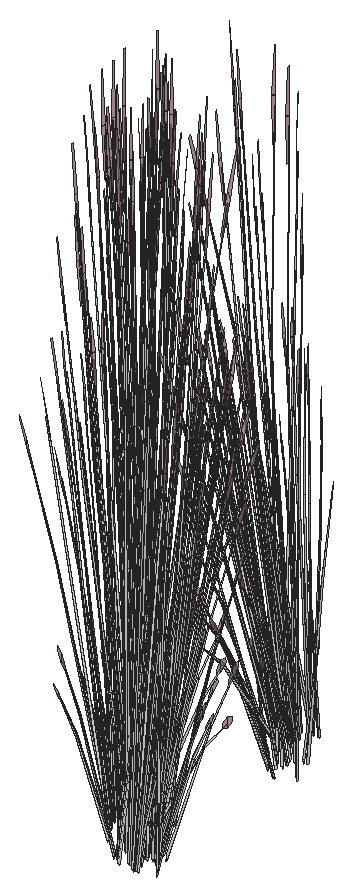
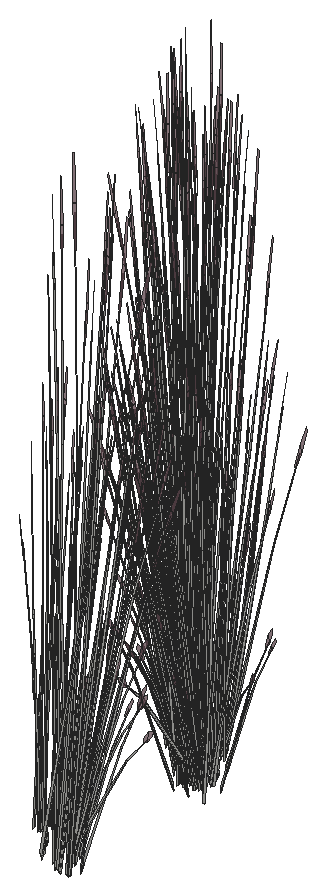
# SketchUp Ruby script. Lengths in inches.
U = 1.inch
M = Sketchup.active_model
def pt(a) = Geom::Point3d.new(a.map { |v| v * U })
def face(e, loops, mat)
  f = e.add_face(loops[0].map { |a| pt(a) })
  loops[1..].each { |l| e.add_face(l.map { |a| pt(a) }).erase! }
  f.material = f.back_material = mat if mat
  f
end
# faces: each face lists its corners as indices into pts; further lists are holes
def faces(e, pts, list, mat = nil) = list.each { |f| face(e, (f[0].is_a?(Array) ? f : [f]).map { |l| l.map { |i| pts[i] } }, mat) }
# xy, xz, yz: faces in a plane at the given z, y or x. An outline is a flat list of corners, or four numbers for a rectangle; further outlines are holes
def ring(l) = l.size == 4 ? [[l[0], l[1]], [l[2], l[1]], [l[2], l[3]], [l[0], l[3]]] : l.each_slice(2).to_a
def flat(e, list, mat, &to3) = list.each { |f| face(e, (f[0].is_a?(Array) ? f : [f]).map { |l| ring(l).map { |u, v| to3.(u, v) } }, mat) }
def xy(e, z, list, mat = nil) = flat(e, list, mat) { |x, y| [x, y, z] }
def xz(e, y, list, mat = nil) = flat(e, list, mat) { |x, z| [x, y, z] }
def yz(e, x, list, mat = nil) = flat(e, list, mat) { |y, z| [x, y, z] }
def lines(e, pts, list) = list.each { |a, b| e.add_line(pt(pts[a]), pt(pts[b])) }
# prism: a flat outline (further loops are holes) pulled along v
def prism(e, loops, v, mat = nil)
  f = face(e, loops, mat); d = Geom::Vector3d.new(v.map { |x| x * U })
  f.pushpull(f.normal.samedirection?(d) ? d.length : -d.length)
end
def box(e, o, s, mat = nil) = prism(e, [[o, [o[0] + s[0], o[1], o[2]], [o[0] + s[0], o[1] + s[1], o[2]], [o[0], o[1] + s[1], o[2]]]], [0, 0, s[2]], mat)
def at(x, y, z, deg = 0) = Geom::Transformation.translation(pt([x, y, z])) * Geom::Transformation.rotation(ORIGIN, Z_AXIS, deg.degrees)
def axes(o, x, y, z) = Geom::Transformation.new([*x, 0, *y, 0, *z, 0, *pt(o).to_a, 1])
def part(name) = M.definitions.add(name)
# library, detail: a bought-in or finely detailed component or shape, given as its bounding box
def library(name, o, s) = part(name).tap { |d| box(d.entities, o, s) }
def detail(e, o, s) = box(e.add_group.entities, o, s)
def put(e, d, t, mat = nil) = e.add_instance(d, t).tap { |i| i.material = mat if mat }
def group(e, t, mat = nil) = e.add_group.tap { |g| g.transformation = t; g.material = mat if mat }.entities
root = M.entities
M.materials.add("LightPink_Translucent").color = [144, 107, 117]
M.materials["LightPink_Translucent"].alpha = 0.75
c1 = part("blade")
p = [[2.15,0.21,22],[0,0.17,0],[0.09,0.45,0],[2.18,0.31,22],[2.29,0.31,22],[0.38,0.45,0],
  [2.48,0.24,33],[2.49,0.24,33],[2.48,0.22,33]]
faces(c1.entities,p,[[0,1,2,3],[4,5,2,3],[6,3,4,7],[8,0,3,6]])
c2 = part("seeds")
p = [[0.3,-0.1,1.38],[-0.01,-0.03,1.59],[-0.01,-0.03,0.03],[0.14,-0.07,-0.07],[0.29,-0.03,3],[0.15,0.01,3.11]]
faces(c2.entities,p,[[0,1,2,3],[1,0,4,5]],"LightPink_Translucent")
c3 = part("blade with seeds")
put(c3.entities,c1,at(0,0,0))
put(c3.entities,c2,axes([2.4,0.25,30.99],[1.5799,-0.05474,1.17369],[-0.12525,1.92788,0.29478],[-0.07173,-0.02425,1.56792]))
put(root,c3,axes([329.78,500.37,1402.68],[-0.25628,0.30892,-0.51099],[-0.22444,-0.32634,-0.3958],[-0.13021,-0.047,0.97773]))
put(root,c3,axes([329.97,500.23,1403.05],[0.20082,0.29199,0.35414],[-0.2293,0.2764,-0.4572],[-0.1165,-0.04206,0.87481]))
put(root,c3,axes([329.2,500.78,1400.77],[0.22533,-0.03337,1.1486],[-0.14293,0.29403,0.84392],[-0.11135,-0.04411,0.25299]))
put(root,c3,axes([330.79,501.05,1400.72],[-0.38326,0.02879,0.44739],[-0.03466,-0.47788,-0.21531],[0.06861,-0.04843,1.43643]))
put(root,c3,axes([329.91,500.05,1403.03],[-0.0189,0.47427,-0.1216],[-0.35781,-0.01296,-0.67495],[-0.13781,-0.03295,1.02557]))
put(root,c3,axes([329.8,501.4,1400.48],[0,0.46636,0.49651],[-0.39487,0,0],[0,-0.10622,1.57504]))
put(root,c3,axes([332.59,501.87,1403.03],[-0.17758,-0.42229,-0.1216],[0.31518,-0.20752,-0.67495],[0.13282,-0.05572,1.02557]))
put(root,c3,axes([332.57,501.51,1402.68],[0.09562,-0.42421,-0.51099],[0.32782,0.1454,-0.3958],[0.13199,-0.0389,0.97773]))
put(root,c3,axes([332.06,499.78,1400.375],[0.22066,-0.46731,0],[0.36918,0.26061,-0.51607],[0.08408,0.05936,1.63711]))
put(root,c3,axes([329.46,500.7,1401.875],[0.14639,-0.01056,1.71376],[-0.09712,0.45778,0.13857],[-0.20862,-0.02831,0.73262]))
put(root,c3,axes([330.73,501.78,1400.21],[-0.21202,-0.39143,-0.44739],[0.32115,-0.27564,0.21531],[-0.06861,-0.04843,1.43643]))
put(root,c3,axes([330.78,501.23,1400.36],[0.15345,0.52148,0.45755],[-0.43845,0.18134,0.17955],[0.00536,-0.09582,1.58856]))
put(root,c3,axes([332.92,501.625,1399.98],[-0.22732,0.05597,1.41583],[-0.03618,-0.44548,0.08104],[0.15921,-0.06743,0.80566]))
put(root,c3,axes([333.34,501.23,1400.26],[-0.21881,-0.29821,-0.06488],[0.23965,-0.27324,-0.29416],[0.0679,-0.01924,0.97024]))
put(root,c3,axes([330.7,501.64,1400.72],[-0.17124,0.42022,0.44739],[-0.35581,-0.20224,-0.21531],[0,-0.09687,1.43643]))
put(root,c3,axes([331.33,501.27,1400.21],[0,-0.53961,0],[0.44133,0,0],[0,0,1.79456]))
put(root,c3,axes([331.87,500.02,1400.48],[-0.33032,-0.23318,0.49651],[0.19744,-0.41812,0],[0.07523,0.05311,1.57504]))
put(root,c3,axes([332.51,501.66,1402.98],[0.31014,-0.20596,-0.71045],[0.17284,0.42397,0.08574],[0.14985,-0.04816,1.00501]))
put(root,c3,axes([330.54,501.93,1400.06],[-0.36714,-0.07646,-0.62353],[0.07747,-0.47163,-0.16365],[-0.10956,-0.05715,1.37633]))
put(root,c3,axes([331.12,500.93,1400.36],[-0.29264,0.42323,0.45755],[-0.34767,-0.3736,0.17955],[0.07055,-0.04224,1.58856]))
put(root,c3,axes([331.44,501.6875,1400.3],[-0.32829,-0.4014,-0.06131],[0.32849,-0.40164,0],[-0.01146,-0.01402,1.75571]))
put(root,c3,axes([330.61,500.23,1400.47],[-0.10196,0.46348,0.17642],[-0.3731,-0.13116,0.35086],[0.06445,-0.00226,1.60407]))
put(root,c3,axes([332.47,501.74,1403.05],[-0.29332,-0.1301,0.35414],[0.08555,-0.37955,-0.4572],[0.11809,-0.0348,0.87481]))
put(root,c3,axes([329.4,501.05,1402.73],[0.09971,-0.42522,0.48003],[0.32782,0.1454,0.3958],[-0.12892,0.02555,0.9933]))
put(root,c3,axes([330.46,500.61,1399.59],[-0.3474,0.18671,1.28929],[-0.11057,-0.53572,0.50096],[0.21332,0.00891,1.46642]))
put(root,c3,axes([331.39,500.75,1400.62],[0.06809,-0.4162,0.1448],[0.33266,0.07225,-0.41347],[0.06054,0.04274,1.26744]))
put(root,c3,axes([329.37,500.9375,1402.73],[-0.12963,-0.31798,0.0643],[0.23638,-0.15564,0.50621],[-0.1042,0.03071,0.77189]))
put(root,c3,axes([330.82,501.74,1400.36],[0.44609,0.09826,0.45755],[-0.09078,0.55493,0.17955],[-0.06519,-0.05359,1.58856]))
put(root,c3,axes([333.17,501.33,1399.49],[-0.01845,-0.0708,1.76342],[0.12793,-0.41416,-0.26939],[0.12905,-0.00596,0.30037]))
put(root,c3,axes([329.36,501.26,1399.49],[0.00895,0.0735,1.76342],[-0.18044,0.38382,-0.26939],[-0.12817,-0.01935,0.30037]))
put(root,c3,axes([331.25,500.86,1400.72],[-0.21202,-0.39143,0.44739],[0.32115,-0.27564,-0.21531],[0.06861,0.04843,1.43643]))
put(root,c3,axes([330.15,502.65,1400.03],[-0.08291,-0.40636,-0.30978],[0.32928,-0.11539,0.30978],[-0.06638,-0.04686,1.38974]))
put(root,c3,axes([330.58,502.625,1400.47],[0.37926,-0.12378,0.17642],[0.09365,0.46065,0.35086],[-0.03382,-0.06712,1.60407]))
put(root,c3,axes([331.36,500.88,1400.67],[0.35635,-0.30962,-0.29095],[0.23697,0.43749,-0.50002],[0.08792,0.04443,1.59708]))
put(root,c3,axes([332.78,501.7,1402.53],[0.29332,0.1301,-0.35414],[-0.08555,0.37955,0.4572],[0.11809,-0.0348,0.87481]))
put(root,c3,axes([330.0625,502.82,1400.02],[-0.33032,-0.23318,-0.49651],[0.19744,-0.41812,0],[-0.07523,-0.05311,1.57504]))
put(root,c3,axes([332.26,500.0625,1400.02],[0.33032,0.23318,-0.49651],[-0.19744,0.41812,0],[0.07523,0.05311,1.57504]))
put(root,c3,axes([329.33,501.1,1402.53],[-0.29332,-0.1301,-0.35414],[0.08555,-0.37955,0.4572],[-0.11809,0.0348,0.87481]))
put(root,c3,axes([331.63,501.39,1400.21],[0.39487,0,0],[0,0.48281,0],[0,0,1.78407]))
put(root,c3,axes([330.96,502,1400.67],[-0.35635,0.30962,-0.29095],[-0.23697,-0.43749,-0.50002],[-0.08792,-0.04443,1.59708]))
put(root,c3,axes([331.74,500.26,1400.47],[-0.37926,0.12378,0.17642],[-0.09365,-0.46065,0.35086],[0.03382,0.06712,1.60407]))
put(root,c3,axes([331.98,501.23,1401.875],[-0.14639,0.01056,1.71376],[0.09712,-0.45778,0.13857],[0.20862,0.02831,0.73262]))
put(root,c3,axes([332.17,500.23,1400.03],[0.08291,0.40636,-0.30978],[-0.32928,0.11539,0.30978],[0.06638,0.04686,1.38974]))
put(root,c3,axes([332.73,501.86,1402.73],[0.12963,0.31798,0.0643],[-0.23638,0.15564,0.50621],[0.1042,-0.03071,0.77189]))
put(root,c3,axes([331.5,501.15,1400.38],[-0.44609,-0.09826,0.49198],[0.09078,-0.55493,0.19306],[0.06519,0.05359,1.70813]))
put(root,c3,axes([332.71,501.75,1402.73],[-0.09971,0.42522,0.48003],[-0.32782,-0.1454,0.3958],[0.12892,-0.02555,0.9933]))
put(root,c3,axes([331.15,502.52,1400.2],[-0.11516,-0.40207,0],[0.32884,-0.1408,0],[0,0,1.54371]))
put(root,c3,axes([330.93,502.13,1400.62],[-0.06809,0.4162,0.1448],[-0.33266,-0.07225,-0.41347],[-0.06054,-0.04274,1.26744]))
put(root,c3,axes([329.64,501.05,1403.05],[0.29332,0.1301,0.35414],[-0.08555,0.37955,-0.4572],[-0.11809,0.0348,0.87481]))
put(root,c3,axes([331.58,502.46,1400.18],[0.37054,-0.15823,-0.19198],[0.1302,0.45581,0.00008],[0.0409,-0.01749,1.73897]))
put(root,c3,axes([331.71,502.65,1400.47],[0.10196,-0.46348,0.17642],[0.3731,0.13116,0.35086],[-0.06445,0.00226,1.60407]))
put(root,c3,axes([331.62,501.6,1400.21],[0.24637,0.30123,0],[-0.24637,0.30123,0],[0,0,1.69266]))
put(root,c3,axes([330.22,501.03,1401.34],[0.10032,-0.06746,1.77064],[0.0346,0.47103,0.13857],[-0.2173,0.0625,0.63284]))
put(root,c3,axes([332.29,501.47,1400.47],[-0.2773,-0.3397,0.17642],[0.27945,-0.32949,0.35086],[-0.03063,0.06937,1.60407]))
put(root,c3,axes([331.78,500.95,1400.06],[0.36714,0.07646,-0.62353],[-0.07747,0.47163,-0.16365],[0.10956,0.05715,1.37633]))
put(root,c3,axes([333.4,501.78,1400.77],[-0.21807,0.07699,1.1486],[0.10265,-0.31819,0.84392],[0.11568,0.02177,0.25299]))
put(root,c3,axes([331.07,502.7,1400.2],[-0.35581,-0.20937,0],[0.17124,-0.43505,0],[0,0,1.62707]))
put(root,c3,axes([331.36,502.14,1400.46],[-0.34464,-0.37536,-0.25192],[0.29,-0.42149,0.5513],[-0.0928,0.04391,1.68216]))
put(root,c3,axes([330.45,502.86,1400.48],[0.33032,0.23318,0.49651],[-0.19744,0.41812,0],[-0.07523,-0.05311,1.57504]))
put(root,c3,axes([331.62,501.25,1400.72],[0.17124,-0.42022,0.44739],[0.35581,0.20224,-0.21531],[0,0.09687,1.43643]))
put(root,c3,axes([333.3,503.125,1402.71],[-0.03191,-0.04083,1.77383],[0.06981,-0.43764,-0.16761],[0.12571,-0.02796,0.31391]))
put(root,c3,axes([329.14,501.35,1402.72],[-0.05763,0.06055,1.74944],[0.0049,0.44239,-0.27667],[-0.13211,0.05753,0.14031]))
put(root,c3,axes([331.55,501.49,1400.29],[0,0.53934,-0.05637],[-0.44133,0,0],[0,0.01695,1.79368]))
put(root,c3,axes([329.53,501.29,1402.68],[-0.09562,0.42421,-0.51099],[-0.32782,-0.1454,-0.3958],[-0.13199,0.0389,0.97773]))
put(root,c3,axes([329.51,500.93,1403.03],[0.17758,0.42229,-0.1216],[-0.31518,0.20752,-0.67495],[-0.13282,0.05572,1.02557]))
put(root,c3,axes([331.58,501.1,1400.21],[0.21202,0.39143,-0.44739],[-0.32115,0.27564,0.21531],[0.06861,0.04843,1.43643]))
put(root,c3,axes([333.02,502.76,1401.93],[-0.06755,-0.39203,-0.03492],[0.31928,-0.09013,-0.15832],[0.06667,0.02485,0.52218]))
put(root,c3,axes([330.26,503.1,1400.375],[-0.22066,0.46731,0],[-0.36918,-0.26061,-0.51607],[-0.08408,-0.05936,1.63711]))
put(root,c3,axes([332.19,502.75,1403.03],[0.0189,-0.47427,-0.1216],[0.35781,0.01296,-0.67495],[0.13781,0.03295,1.02557]))
put(root,c3,axes([332.52,501.48,1400.48],[0,-0.46636,0.49651],[0.39487,0,0],[0,0.10622,1.57504]))
put(root,c3,axes([331.53,501.83,1400.72],[0.38326,-0.02879,0.44739],[0.03466,0.47788,-0.21531],[-0.06861,0.04843,1.43643]))
put(root,c3,axes([331.77,501.34,1400.62],[0.32884,-0.136,0.1448],[0.11516,0.38837,-0.41347],[0,0.08547,1.26744]))
put(root,c3,axes([332.14,502.5625,1403.05],[-0.20082,-0.29199,0.35414],[0.2293,-0.2764,-0.4572],[0.1165,0.04206,0.87481]))
put(root,c3,axes([331.1875,502.06,1400.21],[-0.38326,0.02879,-0.44739],[-0.03466,-0.47788,0.21531],[-0.06861,0.04843,1.43643]))
put(root,c3,axes([332.99,502.29,1400.59],[-0.085,-0.1147,1.43002],[0.1106,-0.37943,-0.30754],[0.17198,0.0514,0.61141]))
put(root,c3,axes([331.47,502.71,1400.2],[0.35581,0.20937,0],[-0.17124,0.43505,0],[0,0,1.74954]))
put(root,c3,axes([332.5,502.46,1402.72],[0.07571,-0.00789,1.74944],[0.20767,-0.36231,-0.27667],[0.13467,0.04783,0.14031]))
put(root,c3,axes([331.61,503.17,1400.19],[-0.21791,-0.46895,-0.05142],[0.36918,-0.26061,0.51607],[-0.09097,0.04465,1.6363]))
put(root,c3,axes([331.53,502.03,1400.62],[0.26075,0.2802,0.1448],[-0.2175,0.31612,-0.41347],[-0.06054,0.04274,1.26744]))
put(root,c3,axes([329.47,502.11,1402.73],[-0.08753,-0.42921,0.48003],[0.34336,-0.07449,0.3958],[-0.1012,0.10094,0.9933]))
put(root,c3,axes([329.41,502.03,1402.73],[-0.2423,-0.19613,0.0643],[0.14107,-0.2793,0.50621],[-0.07768,0.0903,0.77189]))
put(root,c3,axes([329.52,501.51,1401.875],[0.12246,-0.09864,1.71376],[0.1031,0.45582,0.13857],[-0.19225,0.10302,0.73262]))
put(root,c3,axes([332.21,502.52,1402.98],[0.35281,0.01123,-0.71045],[-0.0237,0.47284,0.08574],[0.14947,0.0499,1.00501]))
put(root,c3,axes([331.8125,502.9,1400.48],[0.33032,-0.23318,0.49651],[0.19744,0.41812,0],[-0.07523,0.05311,1.57504]))
put(root,c3,axes([331.34,502.53,1400.29],[0.15345,0.53576,-0.06012],[-0.43845,0.18773,0],[0.00536,0.01871,1.72173]))
put(root,c3,axes([331.51,503.11,1400.03],[-0.32928,-0.11539,-0.30978],[0.08291,-0.40636,0.30978],[-0.06638,0.04686,1.38974]))
put(root,c3,axes([329.14,502.28,1400.59],[0.12266,0.03828,1.43002],[0.07906,0.39104,-0.30754],[-0.16661,0.0732,0.61141]))
put(root,c3,axes([329.6875,501.96,1403.05],[0.30722,-0.06665,0.35414],[0.08112,0.381,-0.4572],[-0.08804,0.10234,0.87481]))
put(root,c3,axes([332.78,501.56,1400.375],[0.44133,0,0],[0,0.52122,-0.51607],[0,0.11871,1.63711]))
put(root,c3,axes([328.5,501.8,1402.71],[0.04504,0.01251,1.77383],[0.13934,0.41205,-0.16761],[-0.0922,0.10815,0.31391]))
put(root,c3,axes([332.61,501.83,1400.2],[-0.44111,-0.00373,-0.04976],[0,-0.52122,0.49943],[-0.01386,0.11865,1.58352]))
put(root,c3,axes([331.65,501.375,1400.67],[0.39748,0.22252,-0.29095],[-0.19139,0.46966,-0.50002],[0.01249,0.11531,1.59708]))
put(root,c3,axes([328.88,503.1,1400.77],[0.14709,-0.21136,1.1486],[0.05804,0.3346,0.84392],[-0.1063,0.05991,0.25299]))
put(root,c3,axes([332.42,502.71,1402.53],[0.20082,0.29199,-0.35414],[-0.2293,0.2764,0.4572],[0.1165,0.04206,0.87481]))
put(root,c3,axes([332.52,501.9,1400.03],[-0.24637,0.29097,-0.30978],[-0.24637,-0.29097,0.30978],[0,0.09372,1.38974]))
put(root,c3,axes([331.46,501.93,1400.67],[0.04113,0.53214,-0.29095],[-0.42835,0.03218,-0.50002],[-0.07543,0.07088,1.59708]))
put(root,c3,axes([332.32,502.83,1402.73],[-0.01777,0.35463,0.0643],[-0.26836,-0.00972,0.50621],[0.1028,0.03711,0.77189]))
put(root,c3,axes([331.61,501.72,1400.21],[-0.17124,0.42022,-0.44739],[-0.35581,-0.20224,0.21531],[0,0.09687,1.43643]))
put(root,c3,axes([329.43,502.19,1402.53],[-0.30722,0.06665,-0.35414],[-0.08112,-0.381,0.4572],[-0.08804,0.10234,0.87481]))
put(root,c3,axes([332.34,502.71,1402.73],[-0.26024,0.30729,0.48003],[-0.22444,-0.32634,0.3958],[0.1221,0.05668,0.9933]))
put(root,c3,axes([328.99,503.05,1403.65],[0.31145,0.12449,-0.06488],[-0.0958,0.38314,-0.29416],[-0.05094,0.05817,0.97024]))
put(root,c3,axes([331.2,502.34,1400.06],[-0.23773,0.35053,-0.62353],[-0.29532,-0.31785,-0.16365],[-0.09526,0.08744,1.37633]))
put(root,c3,axes([331.52,503.07,1403.05],[-0.05451,-0.37564,0.35414],[0.31161,-0.09919,-0.4572],[0.0837,0.10765,0.87481]))
put(root,c3,axes([331.62,502.93,1400.33],[0.44186,0.15158,0.30756],[-0.11054,0.54181,-0.36492],[-0.07313,0.06781,1.64885]))
put(root,c3,axes([331.59,503.29,1400.02],[-0.33032,0.23318,-0.49651],[-0.19744,-0.41812,0],[-0.07523,0.05311,1.57504]))
put(root,c3,axes([332.6875,501.91,1400.02],[0,0.46636,-0.49651],[-0.39487,0,0],[0,0.10622,1.57504]))
put(root,c3,axes([331.7,501.97,1401.875],[-0.1311,-0.08035,1.71376],[0.27131,-0.33708,0.13857],[0.16909,0.15206,0.73262]))
put(root,c3,axes([331.72,500.91,1402.47],[-0.30498,-0.24231,1.38283],[0.32203,-0.37727,0.59665],[0.0984,0.22736,1.33663]))
put(root,c3,axes([329.53,501.93,1403.03],[0.32648,0.25715,-0.1216],[-0.18809,0.3724,-0.67495],[-0.09224,0.12945,1.02557]))
put(root,c3,axes([332.18,502.88,1400.77],[-0.19872,-0.13409,1.1486],[0.2566,-0.13625,0.84392],[0.06921,0.11541,0.25299]))
put(root,c3,axes([331.49,503.26,1403.03],[0.21031,-0.39918,-0.1216],[0.30457,0.22997,-0.67495],[0.10587,0.11278,1.02557]))
put(root,c3,axes([329.97,501.82,1401.875],[0.08815,-0.14329,1.71376],[0.22258,0.38678,0.13857],[-0.15267,0.17614,0.73262]))
put(root,c3,axes([329.6875,502.23,1402.68],[0.09067,0.42583,-0.51099],[-0.34336,0.07449,-0.3958],[-0.0984,0.11438,0.97773]))
put(root,c3,axes([330.1,502.72,1403.05],[0.23881,-0.24554,0.35414],[0.22606,0.28036,-0.4572],[-0.0344,0.14245,0.87481]))
put(root,c3,axes([331.89,503.22,1400.375],[0.22066,0.46731,0],[-0.36918,0.26061,-0.51607],[-0.08408,0.05936,1.63711]))
put(root,c3,axes([331.21,503.59,1402.71],[0.00104,-0.05646,1.77383],[0.30246,-0.2491,-0.16761],[0.10506,0.08891,0.31391]))
put(root,c3,axes([332.24,503.38,1399.49],[0.02571,-0.06733,1.76342],[0.32373,-0.19829,-0.26939],[0.09815,0.10263,0.30037]))
put(root,c3,axes([331.7,501.37,1400.84],[-0.00964,-0.43909,1.41272],[0.43635,0.11382,0.59816],[-0.1032,0.24027,1.3335]))
put(root,c3,axes([331.8125,501.85,1400.09],[0.12941,0.42699,-0.69212],[-0.37279,0.15378,-0.18165],[0.0143,0.14459,1.52773]))
put(root,c3,axes([329.88,502.95,1402.73],[-0.29004,-0.02173,0.0643],[0.00795,-0.32812,0.50621],[-0.03035,0.12569,0.77189]))
put(root,c3,axes([329.27,503.32,1399.49],[0.04734,0.04659,1.76342],[0.08027,0.4317,-0.26939],[-0.10492,0.09206,0.30037]))
put(root,c3,axes([329.98,502.98,1402.73],[-0.25132,-0.3182,0.48003],[0.2669,-0.27442,0.3958],[-0.04636,0.14929,0.9933]))
put(root,c3,axes([331.74,503.06,1402.68],[0.34827,-0.11086,-0.51099],[0.06092,0.41983,-0.3958],[0.09354,0.12031,0.97773]))
put(root,c3,axes([330.77,503.13,1403.05],[0.1064,-0.35863,0.35414],[0.31043,0.1046,-0.4572],[0.02846,0.14439,0.87481]))
put(root,c3,axes([332.22,503.49,1400.67],[-0.22633,-0.01463,1.0506],[0.14947,-0.31064,0.58006],[0.08941,0.11036,0.8241]))
put(root,c3,axes([331.56,503.41,1402.73],[-0.16041,0.29625,0.0643],[-0.22843,-0.17248,0.50621],[0.07385,0.09498,0.77189]))
put(root,c3,axes([331.1875,504.41,1403.65],[0.2439,-0.26754,-0.06488],[0.22348,0.29302,-0.29416],[0.01573,0.08303,0.97024]))
put(root,c3,axes([331.63,503.33,1402.73],[-0.35104,0.10702,0.48003],[-0.06092,-0.41983,0.3958],[0.08256,0.12373,0.9933]))
put(root,c3,axes([329.9,502.17,1401.875],[0.06572,-0.16029,1.71376],[0.27569,0.33172,0.13857],[-0.12437,0.20675,0.73262]))
put(root,c3,axes([331.48,502.74,1400.59],[0.00623,-0.15459,1.43002],[0.29764,-0.17268,-0.30754],[0.09188,0.18503,0.61141]))
put(root,c3,axes([330.67,503.45,1402.73],[-0.26007,0.1585,0.0643],[-0.12729,-0.28902,0.50621],[0.02512,0.1274,0.77189]))
put(root,c3,axes([329.98,503.07,1402.53],[-0.23881,0.24554,-0.35414],[-0.22606,-0.28036,0.4572],[-0.0344,0.14245,0.87481]))
put(root,c3,axes([329.15,503,1402.72],[-0.00877,0.09229,1.74944],[0.24897,0.32105,-0.27667],[-0.06518,0.15182,0.14031]))
put(root,c3,axes([329.95,502.79,1403.4],[0.3879,0.02311,-0.13498],[-0.0106,0.43749,-0.74919],[-0.02694,0.1685,1.13838]))
put(root,c3,axes([330.67,503.28,1403.03],[0.34538,-0.21713,-0.1216],[0.16972,0.38536,-0.67495],[0.04557,0.16239,1.02557]))
put(root,c3,axes([330.77,503.42,1403.0625],[-0.34777,-0.12192,0.53283],[0.11892,-0.40083,0.43934],[0.0209,0.15763,1.10256]))
put(root,c3,axes([330.13,504.03,1400.77],[-0.00913,-0.2773,1.1486],[0.22824,0.19778,0.84392],[-0.04489,0.13217,0.25299]))
put(root,c3,axes([330.73,503.36,1399.49],[0.05712,-0.02538,1.76342],[0.34359,0.13968,-0.26939],[0.01005,0.15742,0.30037]))
put(root,c3,axes([330.21,502.96,1403],[0.25266,0.31335,-0.5672],[-0.2669,0.27442,-0.43934],[-0.03844,0.15921,1.08528]))
put(root,c3,axes([329.9375,503.43,1400.82],[0.32063,-0.08258,0.06507],[0.07371,0.33271,-0.86304],[-0.02033,0.16842,0.7736]))
put(root,c3,axes([330.96,503.26,1402.68],[0.34695,0.11691,-0.51099],[-0.11892,0.40083,-0.3958],[0.03181,0.16138,0.97773]))
put(root,c3,axes([331.16,502.43,1401.875],[-0.08068,-0.14973,1.71376],[0.3728,-0.12606,0.13857],[0.08426,0.23506,0.73262]))
put(root,c3,axes([330.8,503.51,1402.53],[-0.1064,0.35863,-0.35414],[-0.31043,-0.1046,0.4572],[0.02846,0.14439,0.87481]))
put(root,c3,axes([330.13,502.8125,1403.34],[-0.00918,0.43138,-0.7886],[-0.38672,-0.02897,0.09517],[-0.04081,0.18275,1.11556]))
put(root,c3,axes([329.125,503.95,1402.71],[0.04004,-0.02816,1.77383],[0.33095,0.18728,-0.16761],[-0.00778,0.15594,0.31391]))
put(root,c3,axes([330.5,502.51,1401.875],[-0.00864,-0.17899,1.71376],[0.37441,0.11874,0.13857],[-0.02316,0.25508,0.73262]))
put(root,c3,axes([330.84,503.18,1402.98],[0.16845,0.3792,-0.71045],[-0.34676,0.21133,0.08574],[0.03939,0.18322,1.00501]))
put(root,c3,axes([329.86,503.78,1400.59],[0.11138,-0.07357,1.43002],[0.27499,0.22183,-0.30754],[-0.08185,0.19194,0.61141]))
put(root,c3,axes([330.58,504.14,1402.72],[0.04474,0.0751,1.74944],[0.36104,0.0295,-0.27667],[0.03631,0.16562,0.14031]))
put(root,c3,axes([330.01,503.42,1401.36],[0.00775,-0.24075,1.54345],[0.34877,0.12716,0.21329],[-0.03022,0.25658,0.72882]))
put(root,c3,axes([330.27,517.78,1401.875],[0.08068,0.14973,1.71376],[-0.3728,0.12606,0.13857],[-0.08426,-0.23506,0.73262]))
put(root,c3,axes([330.89,516.79,1402.72],[-0.05398,-0.06539,1.74944],[-0.36026,0.04145,-0.27667],[-0.0575,-0.15639,0.14031]))
put(root,c3,axes([331.72,517.5625,1400.59],[-0.10032,0.0944,1.43002],[-0.30046,-0.16522,-0.30754],[0.05569,-0.20547,0.61141]))
put(root,c3,axes([331.27,517.89,1402.98],[-0.16845,-0.3792,-0.71045],[0.34676,-0.21133,0.08574],[-0.03939,-0.18322,1.00501]))
put(root,c3,axes([330.17,517.38,1400.59],[-0.02137,0.15256,1.43002],[-0.31245,0.12771,-0.30754],[-0.07303,-0.19719,0.61141]))
put(root,c3,axes([330.98,517.05,1399.49],[-0.0592,0.0168,1.76342],[-0.32738,-0.18913,-0.26939],[0.00549,-0.15776,0.30037]))
put(root,c3,axes([331.97,518.26,1402.98],[0.00918,-0.43138,-0.71045],[0.38672,0.02897,0.08574],[0.04081,-0.18275,1.00501]))
put(root,c3,axes([332.51,517.59,1402.72],[-0.00341,-0.09282,1.74944],[-0.28775,-0.26825,-0.27667],[0.04449,-0.16261,0.14031]))
put(root,c3,axes([331.3,517.57,1402.53],[0.1064,-0.35863,-0.35414],[0.31043,0.1046,0.4572],[-0.02846,-0.14439,0.87481]))
put(root,c3,axes([331.53,518.04,1401.875],[-0.06572,0.16029,1.71376],[-0.27569,-0.33172,0.13857],[0.12437,-0.20675,0.73262]))
put(root,c3,axes([332.43,517.25,1402.71],[-0.03584,0.03562,1.77383],[-0.35118,-0.12018,-0.16761],[-0.01271,-0.15545,0.31391]))
put(root,c3,axes([331.14,517.8125,1402.68],[-0.34695,-0.11691,-0.51099],[0.11892,-0.40083,-0.3958],[-0.03181,-0.16138,0.97773]))
put(root,c3,axes([331.35,516.81,1400.77],[0.04528,0.27194,1.1486],[-0.25117,-0.15062,0.84392],[0.02703,-0.13924,0.25299]))
put(root,c3,axes([331.89,518.12,1402.68],[-0.25266,-0.31335,-0.51099],[0.2669,-0.27442,-0.3958],[0.03844,-0.15921,0.97773]))
put(root,c3,axes([330.52,516.57,1402.71],[-0.00658,0.0559,1.77383],[-0.32474,0.20287,-0.16761],[-0.09556,-0.1037,0.31391]))
put(root,c3,axes([330.45,517.5625,1403.09],[0.39316,-0.11987,0.53763],[0.06823,0.47021,0.4433],[-0.09247,-0.13858,1.11249]))
put(root,c3,axes([331.34,517.65,1402.73],[0.34777,0.12192,0.48003],[-0.11892,0.40083,0.3958],[-0.0209,-0.15763,0.9933]))
put(root,c3,axes([331.4375,517.79,1403.03],[-0.34538,0.21713,-0.1216],[-0.16972,-0.38536,-0.67495],[-0.04557,-0.16239,1.02557]))
put(root,c3,axes([332.15,518.28,1403.03],[-0.3879,-0.02311,-0.1216],[0.0106,-0.43749,-0.67495],[0.02694,-0.1685,1.02557]))
put(root,c3,axes([332.13,518,1402.53],[0.23881,-0.24554,-0.35414],[0.22606,0.28036,0.4572],[0.0344,-0.14245,0.87481]))
put(root,c3,axes([330.0625,517.14,1400.77],[0.18411,0.16231,1.1486],[-0.26813,0.09757,0.84392],[-0.05737,-0.12474,0.25299]))
put(root,c3,axes([331.43,517.62,1402.73],[0.26007,-0.1585,0.0643],[0.12729,0.28902,0.50621],[-0.02512,-0.1274,0.77189]))
put(root,c3,axes([330.51,518,1402.98],[-0.30095,-0.22541,-0.71045],[0.21388,-0.395,0.08574],[-0.10904,-0.13459,1.00501]))
put(root,c3,axes([330.4,517.7,1402.53],[-0.05451,-0.37564,-0.35414],[0.31161,-0.09919,0.4572],[-0.0837,-0.10765,0.87481]))
put(root,c3,axes([330.54,517.66,1402.73],[0.16041,-0.29625,0.0643],[0.22843,0.17248,0.50621],[-0.07385,-0.09498,0.77189]))
put(root,c3,axes([329.92,517.625,1399.49],[-0.03419,0.06144,1.76342],[-0.3455,0.13246,-0.26939],[-0.08346,-0.12049,0.30037]))
put(root,c3,axes([330.49,519.3125,1400.1],[-0.14494,-0.47823,-0.69835],[0.41752,-0.17223,-0.18329],[-0.01602,-0.16194,1.54149]))
put(root,c3,axes([329.73,518.25,1401.875],[0.1311,0.08035,1.71376],[-0.27131,0.33708,0.13857],[-0.16909,-0.15206,0.73262]))
put(root,c3,axes([332.43,517.85,1399.49],[-0.05283,-0.03674,1.76342],[-0.13569,-0.41045,-0.26939],[0.09154,-0.11138,0.30037]))
put(root,c3,axes([331.33,517.95,1403.05],[-0.1064,0.35863,0.35414],[-0.31043,-0.1046,-0.4572],[-0.02846,-0.14439,0.87481]))
put(root,c3,axes([330.37,518.01,1402.68],[-0.34827,0.11086,-0.51099],[-0.06092,-0.41983,-0.3958],[-0.09354,-0.12031,0.97773]))
put(root,c3,axes([332.125,518.1,1402.73],[0.25132,0.3182,0.48003],[-0.2669,0.27442,0.3958],[0.04636,-0.14929,0.9933]))
put(root,c3,axes([330.61,517.63,1403.43],[-0.23555,0.44708,-0.13619],[-0.34112,-0.25757,-0.75594],[-0.11858,-0.12631,1.14864]))
put(root,c3,axes([332.22,518.125,1402.73],[0.29004,0.02173,0.0643],[-0.00795,0.32812,0.50621],[0.03035,-0.12569,0.77189]))
put(root,c3,axes([332,518.35,1403.05],[-0.23881,0.24554,0.35414],[-0.22606,-0.28036,-0.4572],[0.0344,-0.14245,0.87481]))
put(root,c3,axes([332.42,519.01,1402.98],[0.18436,-0.36797,-0.71045],[0.32306,0.26151,0.08574],[0.11008,-0.13332,1.00501]))
put(root,c3,axes([330.43,517.9375,1400.375],[-0.22066,-0.46731,0],[0.36918,-0.26061,-0.51607],[0.08408,-0.05936,1.63711]))
put(root,c3,axes([332.41,518.84,1402.68],[-0.09067,-0.42583,-0.51099],[0.34336,-0.07449,-0.3958],[0.0984,-0.11438,0.97773]))
put(root,c3,axes([330.92,517.375,1400.13],[-0.2439,0.26754,-0.03893],[-0.22348,-0.29302,-0.17649],[-0.01573,-0.08303,0.58215]))
put(root,c3,axes([329.71,517.51,1402.72],[-0.07594,-0.00329,1.74944],[-0.24177,0.32918,-0.27667],[-0.129,-0.06726,0.14031]))
put(root,c3,axes([332.58,519.14,1403.03],[-0.32648,-0.25715,-0.1216],[0.18809,-0.3724,-0.67495],[0.09224,-0.12945,1.02557]))
put(root,c3,axes([331.23,520.55,1401.33],[0.305,0.18805,1.51261],[-0.29879,0.40513,0.59816],[-0.13384,-0.24012,1.26806]))
put(root,c3,axes([330.59,518.01,1403.05],[0.05451,0.37564,0.35414],[-0.31161,0.09919,-0.4572],[-0.0837,-0.10765,0.87481]))
put(root,c3,axes([329.63,519.25,1400.02],[0,-0.46636,-0.49651],[0.39487,0,0],[0,-0.10622,1.57504]))
put(root,c3,axes([330.73,517.87,1400.02],[0.33032,-0.23318,-0.49651],[0.19744,0.41812,0],[0.07523,-0.05311,1.57504]))
put(root,c3,axes([332.69,518.67,1400.59],[-0.12609,-0.01381,1.43002],[-0.12917,-0.37055,-0.30754],[0.1549,-0.10482,0.61141]))
put(root,c3,axes([329.65,518.25,1403.09],[0.29147,-0.34417,0.53763],[0.25138,0.3655,0.4433],[-0.13675,-0.06349,1.11249]))
put(root,c3,axes([333.38,519.03,1402.71],[-0.0461,-0.00354,1.77383],[-0.19143,-0.37951,-0.16761],[0.07688,-0.12478,0.31391]))
put(root,c3,axes([331.12,518.82,1400.06],[0.23773,-0.35053,-0.62353],[0.29532,0.31785,-0.16365],[0.09526,-0.08744,1.37633]))
put(root,c3,axes([332.84,517.99,1400.77],[-0.11756,0.2374,1.1486],[-0.10105,-0.31895,0.84392],[0.09709,-0.07992,0.25299]))
put(root,c3,axes([332.67,518.88,1402.53],[0.30722,-0.06665,-0.35414],[0.08112,0.381,0.4572],[0.08804,-0.10234,0.87481]))
put(root,c3,axes([329.78,518.25,1402.73],[0.01777,-0.35463,0.0643],[0.26836,0.00972,0.50621],[-0.1028,-0.03711,0.77189]))
put(root,c3,axes([330.71,519.4375,1400.21],[0.17124,-0.42022,-0.44739],[0.35581,0.20224,0.21531],[0,-0.09687,1.43643]))
put(root,c3,axes([329.68,518.36,1402.53],[-0.20082,-0.29199,-0.35414],[0.2293,-0.2764,0.4572],[-0.1165,-0.04206,0.87481]))
put(root,c3,axes([330.86,519.23,1400.67],[-0.04113,-0.53214,-0.29095],[0.42835,-0.03218,-0.50002],[0.07543,-0.07088,1.59708]))
put(root,c3,axes([329.8,519.26,1400.03],[0.24637,-0.29097,-0.30978],[0.24637,0.29097,0.30978],[0,-0.09372,1.38974]))
put(root,c3,axes([329.7,517.86,1400.13],[-0.10181,0.3808,-0.03893],[-0.31336,-0.11714,-0.17649],[-0.04758,-0.06228,0.58215]))
put(root,c3,axes([332.42,519.11,1403.05],[-0.30722,0.06665,0.35414],[-0.08112,-0.381,-0.4572],[0.08804,-0.10234,0.87481]))
put(root,c3,axes([330.67,519.79,1400.67],[-0.39748,-0.22252,-0.29095],[0.19139,-0.46966,-0.50002],[-0.01249,-0.11531,1.59708]))
put(root,c3,axes([329.53,519.6,1400.375],[-0.44133,0,0],[0,-0.52122,-0.51607],[0,-0.11871,1.63711]))
